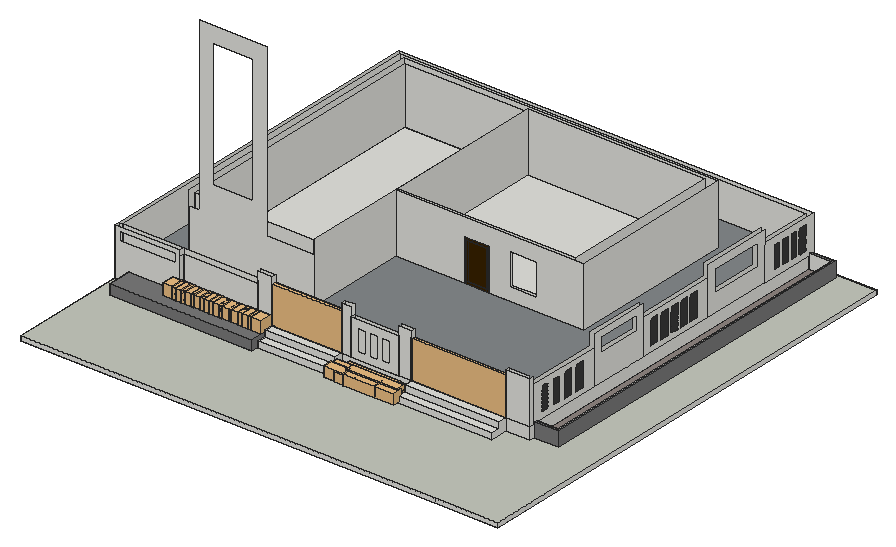
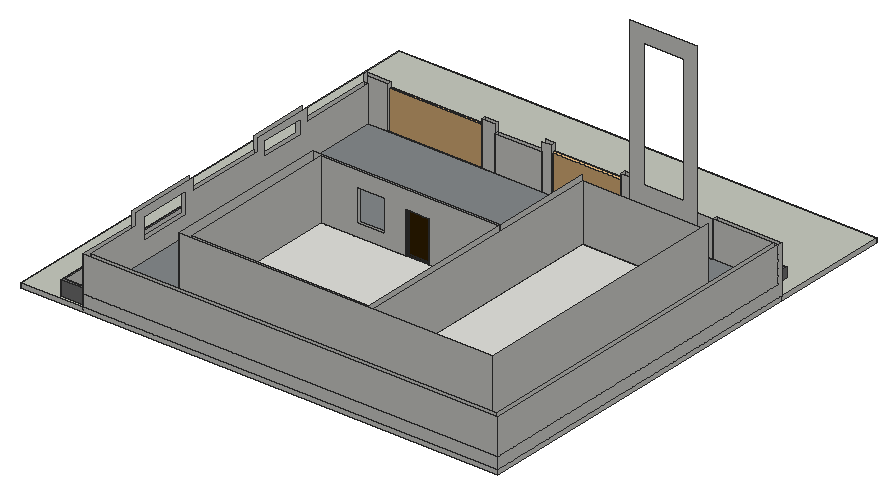
# SketchUp Ruby script. Lengths in inches.
U = 1.inch
M = Sketchup.active_model
def pt(a) = Geom::Point3d.new(a.map { |v| v * U })
def face(e, loops, mat)
  f = e.add_face(loops[0].map { |a| pt(a) })
  loops[1..].each { |l| e.add_face(l.map { |a| pt(a) }).erase! }
  f.material = f.back_material = mat if mat
  f
end
# faces: each face lists its corners as indices into pts; further lists are holes
def faces(e, pts, list, mat = nil) = list.each { |f| face(e, (f[0].is_a?(Array) ? f : [f]).map { |l| l.map { |i| pts[i] } }, mat) }
# xy, xz, yz: faces in a plane at the given z, y or x. An outline is a flat list of corners, or four numbers for a rectangle; further outlines are holes
def ring(l) = l.size == 4 ? [[l[0], l[1]], [l[2], l[1]], [l[2], l[3]], [l[0], l[3]]] : l.each_slice(2).to_a
def flat(e, list, mat, &to3) = list.each { |f| face(e, (f[0].is_a?(Array) ? f : [f]).map { |l| ring(l).map { |u, v| to3.(u, v) } }, mat) }
def xy(e, z, list, mat = nil) = flat(e, list, mat) { |x, y| [x, y, z] }
def xz(e, y, list, mat = nil) = flat(e, list, mat) { |x, z| [x, y, z] }
def yz(e, x, list, mat = nil) = flat(e, list, mat) { |y, z| [x, y, z] }
def lines(e, pts, list) = list.each { |a, b| e.add_line(pt(pts[a]), pt(pts[b])) }
# prism: a flat outline (further loops are holes) pulled along v
def prism(e, loops, v, mat = nil)
  f = face(e, loops, mat); d = Geom::Vector3d.new(v.map { |x| x * U })
  f.pushpull(f.normal.samedirection?(d) ? d.length : -d.length)
end
def box(e, o, s, mat = nil) = prism(e, [[o, [o[0] + s[0], o[1], o[2]], [o[0] + s[0], o[1] + s[1], o[2]], [o[0], o[1] + s[1], o[2]]]], [0, 0, s[2]], mat)
def at(x, y, z, deg = 0) = Geom::Transformation.translation(pt([x, y, z])) * Geom::Transformation.rotation(ORIGIN, Z_AXIS, deg.degrees)
def axes(o, x, y, z) = Geom::Transformation.new([*x, 0, *y, 0, *z, 0, *pt(o).to_a, 1])
def part(name) = M.definitions.add(name)
# library, detail: a bought-in or finely detailed component or shape, given as its bounding box
def library(name, o, s) = part(name).tap { |d| box(d.entities, o, s) }
def detail(e, o, s) = box(e.add_group.entities, o, s)
def put(e, d, t, mat = nil) = e.add_instance(d, t).tap { |i| i.material = mat if mat }
def group(e, t, mat = nil) = e.add_group.tap { |g| g.transformation = t; g.material = mat if mat }.entities
root = M.entities
M.materials.add("[Blacktop Old 01]").color = [132, 136, 139]
M.materials.add("[Color A08]").color = [56, 34, 0]
M.materials.add("[Color M07]").color = [58, 58, 58]
M.materials.add("[Concrete Block Retaining Gray]").color = [121, 121, 121]
M.materials.add("[Groundcover Rock Crushed Multi]").color = [143, 133, 129]
M.materials.add("[Pavers with Grass Herringbone]").color = [197, 201, 190]
M.materials.add("[Pea Gravel]").color = [150, 131, 117]
M.materials.add("[Vegetation Grass Artificial]").color = [98, 140, 74]
c1 = library("chậu cây",[-51.89,-15.59,-1.68],[103.03,17.61,21.35])
c2 = library("plant",[-6.29,-6.78,0],[12.51,14.21,10.3])
c3 = library("Group\#4",[0,0,0],[72.5,6,98.5625])
c4 = library("Group\#5",[0,0,0],[145.875,6,98.5625])
c5 = part("Group\#1")
xy(c5.entities,0,[[0,0,48,2.75]],"[Color A08]")
xy(c5.entities,3.37,[[3.37,0,44.63,2.75]],"[Color A08]")
xy(c5.entities,80.63,[[3.37,0,44.63,2.75]],"[Color A08]")
xy(c5.entities,84,[[0,0,48,2.75]],"[Color A08]")
xz(c5.entities,0,[[[0,0,48,84],[3.37,3.37,44.63,80.63]]],"[Color A08]")
xz(c5.entities,2.75,[[[0,0,48,84],[3.37,3.37,44.63,80.63]],[3.37,3.37,44.63,80.63]],"[Color A08]")
yz(c5.entities,0,[[0,0,2.75,84]],"[Color A08]")
yz(c5.entities,3.37,[[0,3.37,2.75,80.63]],"[Color A08]")
yz(c5.entities,44.63,[[0,3.37,2.75,80.63]],"[Color A08]")
yz(c5.entities,48,[[0,0,2.75,84]],"[Color A08]")
xy(root,0,[[0,163.77,840,402.9],[840,163.77,966.0625,402.9],[0,402.9,840,1122.9],[840,402.9,966.0625,1122.9]])
xy(root,7.89,[[[459.3,358.9,600.55,402.9],[462.25,361.85,597.6,399.94]]])
xy(root,8.625,[[600.66,367.52,791.47,385.21],[600.66,385.21,791.47,402.9]])
xy(root,9,[[[459.3,358.9,600.55,402.9],[462.25,361.85,597.6,399.94]],[318.74,367.52,459.3,385.21],[0,402.9,840,1122.9],[840,413.23,840,418.88,884.9375,418.88,884.9375,1109.45,840,1109.45,840,1115.48,889.9375,1115.48,889.9375,413.23]])
xy(root,9,[[28.56,354.02,317.24,402.9]],"[Concrete Block Retaining Gray]")
xy(root,9,[[840,418.88,884.9375,1109.45]],"[Groundcover Rock Crushed Multi]")
xy(root,9,[[0,163.77,966.0625,163.77,966.0625,1122.9,840,1122.9,840,1115.48,889.9375,1115.48,889.9375,413.23,840,413.23,840,402.9,600.55,402.9,600.55,358.9,459.3,358.9,459.3,367.52,318.74,367.52,318.74,385.21,459.3,385.21,459.3,402.9,317.24,402.9,317.24,354.02,28.56,354.02,28.56,402.9,0,402.9]],"[Pavers with Grass Herringbone]")
xy(root,9,[[462.25,361.85,597.6,399.94]],"[Pea Gravel]")
xy(root,18.8125,[[[459.3,358.9,600.55,402.9],[462.25,361.85,597.6,399.94]]])
xy(root,20.8125,[[600.66,367.52,791.47,385.21]])
xy(root,21.1875,[[318.74,367.52,459.3,385.21]])
xy(root,29.5,[[28.56,354.02,317.24,402.9]],"[Concrete Block Retaining Gray]")
xy(root,33,[[600.66,385.21,791.47,402.9],[132.5,402.9,288.93,411.21],[288.93,402.9,318.78,411.9],[318.78,402.9,459.31,411.9],[459.31,402.9,478.28,411.9],
  [478.28,402.9,575.03,411.9],[575.03,402.9,600.6,411.9],[600.6,402.9,791.47,411.9],[791.47,402.9,840,411.9],[132.5,411.21,288.93,411.9],
  [0,411.9,0,1122.9,840,1122.9,840,411.9,831,411.9,831,1113.9,9,1113.9,9,411.9],[[75.5,496.71,75.5,1041.15,710.3125,1041.15,710.3125,700.96,518.84,700.96,518.84,706.96,689.4375,706.96,689.4375,1035.15,329.75,1035.15,329.75,706.96,470.84,706.96,470.84,700.96,329.75,700.96,329.75,496.71],[81.5,502.71,323.75,1035.15]],[81.5,502.71,323.75,1035.15],[329.75,706.96,689.4375,1035.15]])
xy(root,33,[[[9,411.9,831,1113.9],[75.5,496.71,75.5,1041.15,710.3125,1041.15,710.3125,700.96,518.84,700.96,518.84,706.96,470.84,706.96,470.84,700.96,329.75,700.96,329.75,496.71]]],"[Blacktop Old 01]")
xy(root,33.375,[[318.74,385.21,459.3,402.9]])
xy(root,38.375,[[840,413.23,889.9375,413.23,889.9375,1115.48,840,1115.48,840,1109.45,884.9375,1109.45,884.9375,418.88,840,418.88]],"[Concrete Block Retaining Gray]")
xz(root,163.77,[[0,0,840,9],[840,0,966.0625,9]])
xz(root,354.02,[[28.56,9,317.24,29.5]],"[Concrete Block Retaining Gray]")
xz(root,358.9,[[459.3,7.89,600.55,9]])
xz(root,358.9,[[459.3,9,600.55,18.8125]],"[Concrete Block Retaining Gray]")
xz(root,361.85,[[462.25,7.89,597.6,9]])
xz(root,361.85,[[462.25,9,597.6,18.8125]],"[Vegetation Grass Artificial]")
xz(root,367.52,[[600.66,8.625,791.47,20.8125],[318.74,9,459.3,21.1875]])
xz(root,385.21,[[600.66,20.8125,791.47,33],[318.74,21.1875,459.3,33.375]])
xz(root,399.94,[[462.25,7.89,597.6,9]])
xz(root,399.94,[[462.25,9,597.6,18.8125]],"[Vegetation Grass Artificial]")
xz(root,402.9,[[318.74,7.25,459.3,9],[459.3,7.89,600.55,9],[600.66,8.625,791.47,9],[[0,9,28.56,9,28.56,29.5,317.24,29.5,317.24,9,318.74,9,318.74,33,132.5,33,132.5,105,0,105],[9.54,78.4,123.17,97.78]],[318.74,9,459.3,21.1875],
  [459.3,9,600.55,18.8125],[600.55,9,600.66,9,600.66,33,459.3,33,459.3,18.8125,600.55,18.8125],[600.66,9,791.47,20.8125],[791.47,9,840,33],[600.66,20.8125,791.47,33],
  [318.74,21.1875,459.3,33],[288.93,33,318.74,33,318.74,33.375,318.78,33.375,318.78,122.6875,288.93,122.6875],[318.74,33,318.78,33.375],[318.78,33,459.3,33.375],[459.3,33,459.31,33.375],
  [459.31,33,478.28,124.6875],[[478.28,33,575.03,105],[491.76,47.23,507.7,89.6],[516.07,47.23,532.01,89.6],[540.01,47.23,555.95,89.6]],[575.03,33,600.6,123.125],[791.47,33,840,119.375]])
xz(root,402.9,[[28.56,9,317.24,29.5]],"[Concrete Block Retaining Gray]")
xz(root,411.21,[[132.5,33,288.93,94.09]])
xz(root,411.9,[[0,33,9,105],[9,33,132.5,105],[132.5,33,288.93,105],[288.93,33,318.78,122.6875],[459.31,33,478.28,124.6875],
  [478.28,33,575.03,105],[575.03,33,600.6,123.125],[791.47,33,831,119.375],[831,33,840,105]])
xz(root,413.23,[[840,9,889.9375,38.375]],"[Concrete Block Retaining Gray]")
xz(root,418.88,[[840,9,884.9375,38.375]],"[Vegetation Grass Artificial]")
xz(root,496.71,[[[75.5,33,329.75,33,329.75,125.23,233.4,125.23,233.4,468.42,96.69,468.42,96.69,125.23,75.5,125.23],[122.69,179.43,204.35,436.03]]])
xz(root,502.71,[[81.5,33,323.75,147]])
xz(root,700.96,[[[329.75,33,470.84,33,470.84,117,518.84,117,518.84,33,710.3125,33,710.3125,153,329.75,153],[560.85,58.07,616.42,122.82]]])
xz(root,706.96,[[[329.75,33,329.75,153,689.4375,153,689.4375,33,518.84,33,518.84,117,470.84,117,470.84,33],[560.85,58.07,616.42,122.82]]])
xz(root,1035.15,[[81.5,33,323.75,147],[329.75,33,689.4375,153]])
xz(root,1041.15,[[75.5,33,710.3125,153]])
xz(root,1109.45,[[840,9,884.9375,38.375]])
xz(root,1113.9,[[9,33,831,105]])
xz(root,1115.48,[[840,9,889.9375,38.375]],"[Concrete Block Retaining Gray]")
xz(root,1122.9,[[0,0,840,9],[840,0,966.0625,9],[0,9,840,33],[0,33,840,105]])
yz(root,0,[[163.77,0,402.9,9],[402.9,0,1122.9,9],[402.9,9,402.9,105,411.9,105,411.9,33,1122.9,33,1122.9,9],[411.9,33,1122.9,105]])
yz(root,9,[[411.9,33,1113.9,105]])
yz(root,28.56,[[354.02,9,402.9,29.5]],"[Concrete Block Retaining Gray]")
yz(root,75.5,[[496.71,33,1041.15,153]])
yz(root,81.5,[[502.71,33,1035.15,147]])
yz(root,132.5,[[402.9,33,411.21,94.09],[411.21,33,411.9,33,411.9,105,402.9,105,402.9,94.09,411.21,94.09]])
yz(root,288.93,[[402.9,33,411.21,94.09],[411.21,33,411.21,94.09,402.9,94.09,402.9,105,411.9,105,411.9,33]])
yz(root,317.24,[[354.02,9,402.9,29.5]],"[Concrete Block Retaining Gray]")
yz(root,318.74,[[402.9,7.25,385.21,9,367.52,9,367.52,21.1875,385.21,21.1875,385.21,33.375,402.9,33.375]])
yz(root,318.78,[[402.9,33,411.9,122.6875]])
yz(root,323.75,[[502.71,33,1035.15,147]])
yz(root,329.75,[[496.71,33,700.96,153],[706.96,33,1035.15,153]])
yz(root,459.3,[[402.9,7.25,402.9,7.89,396.46,7.89],[358.9,7.89,367.52,9],[367.52,7.89,385.21,9],[385.21,7.89,385.21,9,396.46,7.89],[396.46,7.89,402.9,7.89,402.9,9,385.21,9],
  [367.52,9,385.21,18.8125],[385.21,9,402.9,18.8125],[367.52,18.8125,402.9,18.8125,402.9,33.375,385.21,33.375,385.21,21.1875,367.52,21.1875]])
yz(root,459.3,[[358.9,9,367.52,18.8125]],"[Concrete Block Retaining Gray]")
yz(root,459.31,[[402.9,33,411.9,124.6875]])
yz(root,462.25,[[361.85,7.89,367.52,9],[367.52,7.89,385.21,9],[385.21,7.89,399.94,9]])
yz(root,462.25,[[361.85,9,399.94,18.8125]],"[Vegetation Grass Artificial]")
yz(root,470.84,[[700.96,33,706.96,117]])
yz(root,478.28,[[402.9,33,411.9,105]])
yz(root,518.84,[[700.96,33,706.96,117]])
yz(root,575.03,[[402.9,33,411.9,105]])
yz(root,597.6,[[361.85,7.89,399.94,9]])
yz(root,597.6,[[361.85,9,399.94,18.8125]],"[Vegetation Grass Artificial]")
yz(root,600.55,[[358.9,7.89,402.9,9]])
yz(root,600.55,[[358.9,9,402.9,18.8125]],"[Concrete Block Retaining Gray]")
yz(root,600.6,[[402.9,33,411.9,123.125]])
yz(root,600.66,[[367.52,8.625,367.52,20.8125,385.21,20.8125,385.21,33,402.9,33,402.9,8.625]])
yz(root,689.4375,[[706.96,33,1035.15,153]])
yz(root,710.3125,[[700.96,33,1041.15,153]])
yz(root,791.47,[[367.52,8.625,402.9,8.625,402.9,33,385.21,33,385.21,20.8125,367.52,20.8125],[402.9,33,411.9,119.375]])
yz(root,831,[[[411.9,33,411.9,105,566.77,105,566.77,129.5,690.36,129.5,690.36,105,853.98,105,853.98,129.5,999.11,129.5,999.11,105,1113.9,105,1113.9,33],[872.22,70.51,980.28,113.38],[582.45,88.15,674.33,117.03]]])
yz(root,840,[[402.9,9,413.23,33],[413.23,9,418.88,33],[418.88,9,1109.45,33],[1109.45,9,1115.48,33],[1115.48,9,1122.9,33],
  [402.9,33,411.9,119.375],[[411.9,33,413.23,33,413.23,38.375,418.88,38.375,418.88,33,566.77,33,566.77,105,411.9,105],[520.34,45.66,536.53,93.98],[492.03,45.66,508.22,93.98],[462.53,45.66,478.72,93.98],[433.47,45.66,449.66,93.98]],[413.23,33,418.88,38.375],[[566.77,33,690.36,129.5],[582.45,88.15,674.33,117.03]],[[690.36,33,853.98,105],[709.66,45.66,725.84,93.98],[735.72,45.66,751.91,93.98],[760.78,45.66,776.97,93.98],[784.91,45.66,801.09,93.98],[808.84,45.66,825.03,93.98]],
  [[853.98,33,999.11,129.5],[872.22,70.51,980.28,113.38]],[[999.11,33,1109.45,33,1109.45,38.375,1115.48,38.375,1115.48,33,1122.9,33,1122.9,105,999.11,105],[1085.5,44.4,1101.69,92.71],[1064.13,44.4,1080.32,92.71],[1042.25,44.4,1058.44,92.71],[1020.5,44.4,1036.69,92.71]],[1109.45,33,1115.48,38.375]])
yz(root,840,[[1020.5,44.4,1036.69,92.71],[1042.25,44.4,1058.44,92.71],[1064.13,44.4,1080.32,92.71],[1085.5,44.4,1101.69,92.71],[433.47,45.66,449.66,93.98],
  [462.53,45.66,478.72,93.98],[492.03,45.66,508.22,93.98],[520.34,45.66,536.53,93.98],[709.66,45.66,725.84,93.98],[735.72,45.66,751.91,93.98],
  [760.78,45.66,776.97,93.98],[784.91,45.66,801.09,93.98],[808.84,45.66,825.03,93.98]],"[Color M07]")
yz(root,884.9375,[[418.88,9,1109.45,38.375]])
yz(root,889.9375,[[413.23,9,1115.48,38.375]],"[Concrete Block Retaining Gray]")
yz(root,966.0625,[[163.77,0,1122.9,9]])
p = [[318.74,385.21,9],[318.74,402.9,7.25],[459.3,402.9,7.25],[459.3,396.46,7.89],[459.3,385.21,9]]
faces(root,p,[[0,1,2,3,4]])
put(root,c1,at(507.4,400.3125,0.84))
put(root,c1,at(524.15,390.24,2.82))
put(root,c1,at(548.11,400.875,3.36))
put(root,c1,at(549.51,396.38,3.36))
put(root,c1,at(539.9,375.1875,5.96))
put(root,c1,at(530.93,373.47,6.35))
put(root,c1,at(529.41,382.85,6.51))
put(root,c1,at(541.97,382.85,6.51))
put(root,c1,at(529.18,397.92,6.99))
put(root,c1,at(511.59,388.63,9))
put(root,c1,at(511.28,373.94,10.68))
put(root,c1,at(551.38,372.56,10.68))
put(root,c1,at(546.64,384.34,12.63))
put(root,c2,axes([243.53,389.15,29.5],[2.1,0,0],[0,1.78,0],[0,0,2.21]))
put(root,c2,axes([224.78,389.15,29.5],[2.1,0,0],[0,1.78,0],[0,0,2.21]))
put(root,c2,axes([206.03,389.15,29.5],[2.1,0,0],[0,1.78,0],[0,0,2.21]))
put(root,c2,axes([187.28,389.15,29.5],[2.1,0,0],[0,1.78,0],[0,0,2.21]))
put(root,c2,axes([168.53,389.15,29.5],[2.1,0,0],[0,1.78,0],[0,0,2.21]))
put(root,c2,axes([149.78,389.15,29.5],[2.1,0,0],[0,1.78,0],[0,0,2.21]))
put(root,c2,axes([131.03,389.15,29.5],[2.1,0,0],[0,1.78,0],[0,0,2.21]))
put(root,c2,axes([263.91,389.15,29.5],[2.1,0,0],[0,1.78,0],[0,0,2.21]))
put(root,c2,axes([282.09,389.15,29.5],[2.1,0,0],[0,1.78,0],[0,0,2.21]))
put(root,c2,axes([302.91,389.15,29.5],[2.1,0,0],[0,1.78,0],[0,0,2.21]))
put(root,c3,axes([318.78,402.9,33],[1.93826,0,0],[0,1,0],[0,0,0.7832]))
put(root,c4,axes([599.82,403.37,33],[1.31538,0,0],[0,0.9212,0],[0,0,0.78302]))
put(root,c5,at(470.84,700.96,33))
